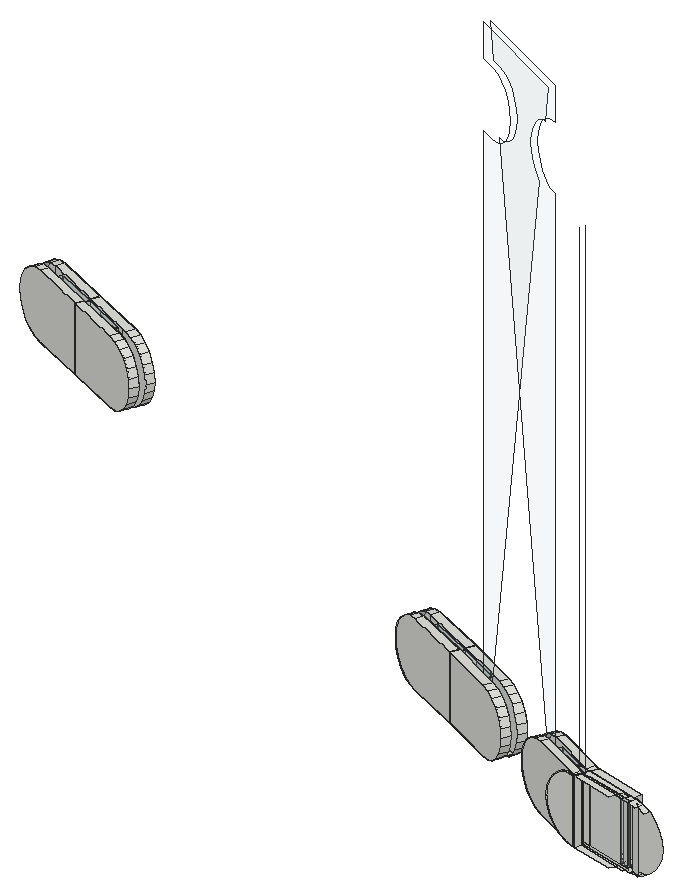
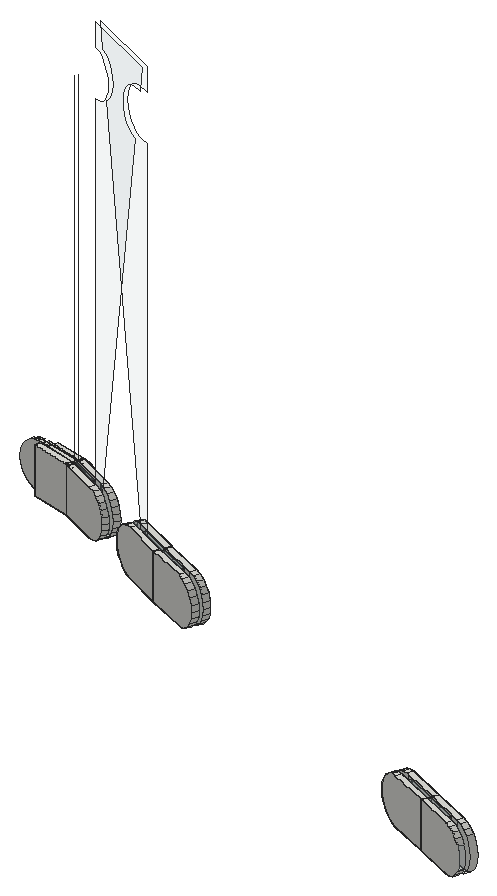
# SketchUp Ruby script. Lengths in inches.
U = 1.inch
M = Sketchup.active_model
def pt(a) = Geom::Point3d.new(a.map { |v| v * U })
def face(e, loops, mat)
  f = e.add_face(loops[0].map { |a| pt(a) })
  loops[1..].each { |l| e.add_face(l.map { |a| pt(a) }).erase! }
  f.material = f.back_material = mat if mat
  f
end
# faces: each face lists its corners as indices into pts; further lists are holes
def faces(e, pts, list, mat = nil) = list.each { |f| face(e, (f[0].is_a?(Array) ? f : [f]).map { |l| l.map { |i| pts[i] } }, mat) }
# xy, xz, yz: faces in a plane at the given z, y or x. An outline is a flat list of corners, or four numbers for a rectangle; further outlines are holes
def ring(l) = l.size == 4 ? [[l[0], l[1]], [l[2], l[1]], [l[2], l[3]], [l[0], l[3]]] : l.each_slice(2).to_a
def flat(e, list, mat, &to3) = list.each { |f| face(e, (f[0].is_a?(Array) ? f : [f]).map { |l| ring(l).map { |u, v| to3.(u, v) } }, mat) }
def xy(e, z, list, mat = nil) = flat(e, list, mat) { |x, y| [x, y, z] }
def xz(e, y, list, mat = nil) = flat(e, list, mat) { |x, z| [x, y, z] }
def yz(e, x, list, mat = nil) = flat(e, list, mat) { |y, z| [x, y, z] }
def lines(e, pts, list) = list.each { |a, b| e.add_line(pt(pts[a]), pt(pts[b])) }
# prism: a flat outline (further loops are holes) pulled along v
def prism(e, loops, v, mat = nil)
  f = face(e, loops, mat); d = Geom::Vector3d.new(v.map { |x| x * U })
  f.pushpull(f.normal.samedirection?(d) ? d.length : -d.length)
end
def box(e, o, s, mat = nil) = prism(e, [[o, [o[0] + s[0], o[1], o[2]], [o[0] + s[0], o[1] + s[1], o[2]], [o[0], o[1] + s[1], o[2]]]], [0, 0, s[2]], mat)
def at(x, y, z, deg = 0) = Geom::Transformation.translation(pt([x, y, z])) * Geom::Transformation.rotation(ORIGIN, Z_AXIS, deg.degrees)
def axes(o, x, y, z) = Geom::Transformation.new([*x, 0, *y, 0, *z, 0, *pt(o).to_a, 1])
def part(name) = M.definitions.add(name)
# library, detail: a bought-in or finely detailed component or shape, given as its bounding box
def library(name, o, s) = part(name).tap { |d| box(d.entities, o, s) }
def detail(e, o, s) = box(e.add_group.entities, o, s)
def put(e, d, t, mat = nil) = e.add_instance(d, t).tap { |i| i.material = mat if mat }
def group(e, t, mat = nil) = e.add_group.tap { |g| g.transformation = t; g.material = mat if mat }.entities
root = M.entities
M.materials.add("Glass_Safety_01").color = [204, 235, 244]
M.materials["Glass_Safety_01"].alpha = 0.1
xy(root,333,[[1023.371,1012.372,1021.983,1012.675,1022.025,1012.868,1023.251,1012.599,1023.444,1012.558],[1023.716,1012.498,1023.444,1012.558,1023.473,1012.632,1023.745,1012.572],[1023.965,1012.524,1023.94,1012.53,1023.97,1012.608,1023.982,1012.603],[1023.94,1012.53,1023.858,1012.548,1023.745,1012.572,1023.787,1012.68,1023.53,1012.78,1023.473,1012.632,1022.042,1012.945,1022.084,1013.137,1022.095,1013.134,1022.105,1013.13,1022.106,1013.132,1023.9,1012.74,1024.007,1012.717,1023.982,1012.603,1023.97,1012.608],[1023.444,1012.558,1023.251,1012.599,1022.025,1012.868,1022.042,1012.945,1023.473,1012.632],
  [1023.745,1012.572,1023.473,1012.632,1023.53,1012.78,1023.787,1012.68],[1021.983,1012.675,1021.876,1012.699,1021.879,1012.714,1021.903,1012.702,1022.02,1012.949,1022.042,1012.945,1022.025,1012.868],[1021.903,1012.702,1021.879,1012.714,1021.935,1012.968,1022.02,1012.949],[1021.879,1012.714,1020.123,1013.542,1020.24,1013.791,1022.021,1012.952,1022.02,1012.949,1021.935,1012.968],[1023.9,1012.74,1022.106,1013.132,1022.222,1013.379,1022.184,1013.397,1023.959,1013.009],
  [1022.105,1013.13,1022.095,1013.134,1022.106,1013.132],[1022.106,1013.132,1022.095,1013.134,1021.983,1013.1875,1022.035,1013.429,1022.184,1013.397,1022.222,1013.379],[1022.095,1013.134,1022.084,1013.137,1021.977,1013.16,1021.983,1013.1875],[1021.983,1013.1875,1020.324,1013.969,1020.442,1014.219,1022.184,1013.397,1022.035,1013.429],[1017.116,1014.96,1015.346,1015.795,1015.456,1016.048,1016.751,1015.437,1016.921,1015.357,1017.234,1015.209],
  [1017.318,1015.387,1016.835,1015.615,1015.537,1016.227,1015.655,1016.476,1017.435,1015.637],[1015.346,1015.795,1015.341,1015.797,1015.336,1015.8,1015.453,1016.049,1015.456,1016.048],[1015.336,1015.8,1013.541,1016.581,1013.651,1016.834,1015.453,1016.049],[1015.535,1016.228,1013.73,1017.014,1013.84,1017.267,1015.645,1016.481],[998.018,1023.342,996.213,1024.128,996.324,1024.38,997.958,1023.669,998.128,1023.594],
  [998.207,1023.775,998.037,1023.849,996.402,1024.561,996.512,1024.814,998.317,1024.028],[996.213,1024.128,994.409,1024.914,994.519,1025.167,996.324,1024.38],[996.402,1024.561,994.597,1025.347,994.707,1025.6,996.512,1024.814]])
xy(root,333.078,[[1023.858,1012.548,1023.745,1012.572,1023.787,1012.68,1023.879,1012.644],[1023.745,1012.572,1023.58,1012.608,1023.622,1012.801,1023.9,1012.74,1023.879,1012.644,1023.787,1012.68],[1023.58,1012.608,1022.319,1012.884,1022.361,1013.076,1023.622,1012.801],[1022.319,1012.884,1022.042,1012.945,1022.063,1013.041,1022.105,1013.13,1022.095,1013.134,1022.361,1013.076],[1022.021,1012.952,1020.597,1013.623,1020.681,1013.801,1022.095,1013.134,1022.084,1013.137,1022.063,1013.041],
  [1022.063,1013.041,1022.084,1013.137,1022.095,1013.134,1022.105,1013.13],[1016.878,1015.377,1016.751,1015.437,1015.456,1016.048,1015.495,1016.138,1015.537,1016.227,1016.835,1015.615,1016.962,1015.555],[1015.455,1016.048,1015.453,1016.049,1015.495,1016.138,1015.456,1016.048],[1015.453,1016.049,1014.012,1016.677,1014.091,1016.857,1015.535,1016.228,1015.495,1016.138],[997.767,1023.752,996.324,1024.38,996.402,1024.561,997.846,1023.932],
  [996.324,1024.38,994.88,1025.009,994.958,1025.19,996.402,1024.561]],"Glass_Safety_01")
xy(root,335.047,[[1023.858,1012.548,1023.879,1012.644,1023.787,1012.68,1023.745,1012.572],[1023.745,1012.572,1023.787,1012.68,1023.879,1012.644,1023.9,1012.74,1023.622,1012.801,1023.58,1012.608],[1023.58,1012.608,1023.622,1012.801,1022.361,1013.076,1022.319,1012.884],[1022.319,1012.884,1022.361,1013.076,1022.095,1013.134,1022.105,1013.13,1022.063,1013.041,1022.042,1012.945],[1022.021,1012.952,1022.063,1013.041,1022.084,1013.137,1022.095,1013.134,1020.681,1013.801,1020.597,1013.623],
  [1022.063,1013.041,1022.105,1013.13,1022.095,1013.134,1022.084,1013.137],[1016.878,1015.377,1016.962,1015.555,1016.835,1015.615,1015.537,1016.227,1015.495,1016.138,1015.456,1016.048,1016.751,1015.437],[1015.455,1016.048,1015.456,1016.048,1015.495,1016.138,1015.453,1016.049],[1015.453,1016.049,1015.495,1016.138,1015.535,1016.228,1014.091,1016.857,1014.012,1016.677],[997.767,1023.752,997.846,1023.932,996.402,1024.561,996.324,1024.38],
  [996.324,1024.38,996.402,1024.561,994.958,1025.19,994.88,1025.009]],"Glass_Safety_01")
xy(root,335.125,[[1023.371,1012.372,1023.444,1012.558,1023.251,1012.599,1022.025,1012.868,1021.983,1012.675],[1023.716,1012.498,1023.745,1012.572,1023.473,1012.632,1023.444,1012.558],[1023.965,1012.524,1023.982,1012.603,1023.97,1012.608,1023.94,1012.53],[1023.94,1012.53,1023.97,1012.608,1023.982,1012.603,1024.007,1012.717,1023.9,1012.74,1022.106,1013.132,1022.105,1013.13,1022.095,1013.134,1022.084,1013.137,1022.042,1012.945,1023.473,1012.632,1023.53,1012.78,1023.787,1012.68,1023.745,1012.572,1023.858,1012.548],[1023.444,1012.558,1023.473,1012.632,1022.042,1012.945,1022.025,1012.868,1023.251,1012.599],
  [1023.745,1012.572,1023.787,1012.68,1023.53,1012.78,1023.473,1012.632],[1021.983,1012.675,1022.025,1012.868,1022.042,1012.945,1022.02,1012.949,1021.903,1012.702,1021.879,1012.714,1021.876,1012.699],[1021.903,1012.702,1022.02,1012.949,1021.935,1012.968,1021.879,1012.714],[1021.879,1012.714,1021.935,1012.968,1022.02,1012.949,1022.021,1012.952,1020.24,1013.791,1020.123,1013.542],[1023.9,1012.74,1023.959,1013.009,1022.184,1013.397,1022.222,1013.379,1022.106,1013.132],
  [1022.105,1013.13,1022.106,1013.132,1022.095,1013.134],[1022.106,1013.132,1022.222,1013.379,1022.184,1013.397,1022.035,1013.429,1021.983,1013.1875,1022.095,1013.134],[1022.095,1013.134,1021.983,1013.1875,1021.977,1013.16,1022.084,1013.137],[1021.983,1013.1875,1022.035,1013.429,1022.184,1013.397,1020.442,1014.219,1020.324,1013.969],[1017.116,1014.96,1017.234,1015.209,1016.751,1015.437,1015.456,1016.048,1015.346,1015.795],
  [1017.318,1015.387,1017.435,1015.637,1015.655,1016.476,1015.537,1016.227,1016.835,1015.615],[1015.346,1015.795,1015.456,1016.048,1015.453,1016.049,1015.336,1015.8,1015.341,1015.797],[1015.336,1015.8,1015.453,1016.049,1013.651,1016.834,1013.541,1016.581],[1015.535,1016.228,1015.645,1016.481,1013.84,1017.267,1013.73,1017.014],[998.018,1023.342,998.128,1023.594,997.958,1023.669,996.324,1024.38,996.213,1024.128],
  [998.207,1023.775,998.317,1024.028,996.512,1024.814,996.402,1024.561,998.037,1023.849],[996.213,1024.128,996.324,1024.38,994.519,1025.167,994.409,1024.914],[996.402,1024.561,996.512,1024.814,994.707,1025.6,994.597,1025.347]])
p = [[1024.276,1012.658,333.036],[1024.526,1012.603,333.142],[1024.484,1012.411,333.142],[1024.234,1012.466,333.036],[1023.745,1012.572,335.125],[1023.858,1012.548,335.125],
  [1023.858,1012.548,335.047],[1023.745,1012.572,335.047],[1023.58,1012.608,335.047],[1023.58,1012.608,333.078],[1023.745,1012.572,333.078],[1023.858,1012.548,333.078],
  [1023.858,1012.548,333],[1023.745,1012.572,333],[1023.473,1012.632,333],[1022.042,1012.945,333],[1022.042,1012.945,333.078],[1022.319,1012.884,333.078],
  [1022.319,1012.884,335.047],[1022.042,1012.945,335.047],[1022.042,1012.945,335.125],[1023.473,1012.632,335.125],[1024.007,1012.717,333],[1023.9,1012.74,333],
  [1023.9,1012.74,333.078],[1023.9,1012.74,335.047],[1023.9,1012.74,335.125],[1024.007,1012.717,335.125],[1024.276,1012.658,335.089],[1024.526,1012.603,334.983],
  [1024.741,1012.556,334.814],[1024.906,1012.52,334.594],[1025.01,1012.497,334.338],[1025.046,1012.49,334.0625],[1025.01,1012.497,333.787],[1024.906,1012.52,333.531],
  [1024.741,1012.556,333.311],[1023.97,1012.608,333],[1023.97,1012.608,333.078],[1023.97,1012.608,335.047],[1023.97,1012.608,335.125],[1023.982,1012.603,335.125],
  [1024.227,1012.508,335.125],[1024.227,1012.508,333],[1023.982,1012.603,333],[1023.965,1012.524,333],[1021.903,1012.702,335.125],[1021.879,1012.714,335.125],
  [1020.123,1013.542,335.125],[1019.874,1013.659,335.089],[1019.642,1013.769,334.983],[1019.443,1013.863,334.814],[1019.29,1013.935,334.594],[1019.194,1013.98,334.338],
  [1019.161,1013.995,334.0625],[1019.194,1013.98,333.787],[1019.29,1013.935,333.531],[1019.443,1013.863,333.311],[1019.642,1013.769,333.142],[1019.874,1013.659,333.036],
  [1020.123,1013.542,333],[1021.879,1012.714,333],[1021.903,1012.702,333],[1021.876,1012.699,333],[1021.983,1012.675,333],[1021.983,1012.675,335.125],
  [1021.876,1012.699,335.125],[1021.607,1012.757,335.089],[1021.357,1012.812,334.983],[1021.141,1012.859,334.814],[1020.976,1012.895,334.594],[1020.873,1012.918,334.338],
  [1020.837,1012.926,334.0625],[1020.873,1012.918,333.787],[1020.976,1012.895,333.531],[1021.141,1012.859,333.311],[1021.357,1012.812,333.142],[1021.607,1012.757,333.036],
  [1021.666,1013.027,333.036],[1021.929,1012.969,333],[1021.935,1012.968,333],[1022.021,1012.952,333],[1022.021,1012.952,333.078],[1022.021,1012.952,335.047],
  [1022.021,1012.952,335.125],[1022.02,1012.949,335.125],[1022.02,1012.949,333],[1022.025,1012.868,335.125],[1022.025,1012.868,333],[1022.095,1013.134,333.078],
  [1022.361,1013.076,333.078],[1023.622,1012.801,333.078],[1022.106,1013.132,333],[1022.095,1013.134,333],[1022.084,1013.137,333],[1022.084,1013.137,333.078],
  [1023.787,1012.68,333.078],[1023.787,1012.68,333],[1023.53,1012.78,333],[1023.53,1012.78,335.125],[1023.787,1012.68,335.125],[1023.787,1012.68,335.047],
  [1023.959,1013.009,333],[1023.959,1013.009,335.125],[1021.415,1013.081,333.142],[1021.935,1012.968,335.125],[1022.063,1013.041,333.078],[1020.24,1013.791,333],
  [1020.24,1013.791,335.125],[1020.597,1013.623,335.047],[1020.597,1013.623,333.078],[1021.666,1013.027,335.089],[1021.929,1012.969,335.125],[1021.2,1013.128,333.311],
  [1021.035,1013.164,333.531],[1020.932,1013.187,333.787],[1020.896,1013.195,334.0625],[1020.932,1013.187,334.338],[1021.035,1013.164,334.594],[1021.2,1013.128,334.814],
  [1021.415,1013.081,334.983],[1022.184,1013.397,335.125],[1022.184,1013.397,333],[1022.035,1013.429,333],[1021.767,1013.488,333.036],[1021.516,1013.543,333.142],
  [1021.301,1013.59,333.311],[1021.136,1013.626,333.531],[1021.032,1013.649,333.787],[1020.997,1013.656,334.0625],[1021.032,1013.649,334.338],[1021.136,1013.626,334.594],
  [1021.301,1013.59,334.814],[1021.516,1013.543,334.983],[1021.767,1013.488,335.089],[1022.035,1013.429,335.125],[1021.983,1013.1875,335.125],[1020.324,1013.969,335.125],
  [1020.324,1013.969,333],[1021.983,1013.1875,333],[1022.105,1013.13,333],[1022.105,1013.13,333.078],[1020.681,1013.801,333.078],[1020.681,1013.801,335.047],
  [1022.095,1013.134,335.047],[1022.105,1013.13,335.047],[1022.105,1013.13,335.125],[1022.095,1013.134,335.125],[1022.084,1013.137,335.125],[1021.977,1013.16,335.125],
  [1021.977,1013.16,333],[1022.084,1013.137,335.047],[1022.222,1013.379,333],[1022.222,1013.379,335.125],[1022.106,1013.132,335.125],[1021.708,1013.219,333.036],
  [1021.97,1013.162,333],[1021.97,1013.162,335.125],[1021.708,1013.219,335.089],[1021.457,1013.274,334.983],[1021.242,1013.321,334.814],[1021.077,1013.357,334.594],
  [1020.974,1013.379,334.338],[1020.938,1013.387,334.0625],[1020.974,1013.379,333.787],[1021.077,1013.357,333.531],[1021.242,1013.321,333.311],[1021.457,1013.274,333.142],
  [1020.442,1014.219,333],[1020.193,1014.336,333.036],[1019.961,1014.445,333.142],[1019.762,1014.539,333.311],[1019.609,1014.611,333.531],[1019.513,1014.657,333.787],
  [1019.481,1014.672,334.0625],[1019.513,1014.657,334.338],[1019.609,1014.611,334.594],[1019.762,1014.539,334.814],[1019.961,1014.445,334.983],[1020.193,1014.336,335.089],
  [1020.442,1014.219,335.125],[1019.992,1013.909,333.036],[1019.76,1014.018,333.142],[1019.992,1013.909,335.089],[1019.76,1014.018,334.983],[1019.561,1014.112,334.814],
  [1019.408,1014.184,334.594],[1019.312,1014.229,334.338],[1019.279,1014.245,334.0625],[1019.312,1014.229,333.787],[1019.408,1014.184,333.531],[1019.561,1014.112,333.311],
  [1019.848,1014.194,334.985],[1020.15,1014.051,333.025],[1020.076,1014.087,335.089],[1020.076,1014.087,333.036],[1019.844,1014.196,333.142],[1019.645,1014.29,333.311],
  [1019.492,1014.362,333.531],[1019.396,1014.407,333.787],[1019.363,1014.423,334.0625],[1019.396,1014.407,334.338],[1019.492,1014.362,334.594],[1019.645,1014.29,334.814],
  [1019.844,1014.196,334.983],[1017.116,1014.96,335.125],[1015.346,1015.795,335.125],[1015.346,1015.795,333],[1017.116,1014.96,333],[1017.365,1014.843,333.036],
  [1017.597,1014.733,333.142],[1017.796,1014.639,333.311],[1017.949,1014.567,333.531],[1018.045,1014.522,333.787],[1018.078,1014.507,334.0625],[1018.045,1014.522,334.338],
  [1017.949,1014.567,334.594],[1017.796,1014.639,334.814],[1017.597,1014.733,334.983],[1017.365,1014.843,335.089],[1017.483,1015.092,333.036],[1017.714,1014.983,333.142],
  [1016.921,1015.357,333],[1017.234,1015.209,333],[1017.914,1014.889,333.311],[1018.066,1014.817,333.531],[1018.162,1014.771,333.787],[1018.195,1014.756,334.0625],
  [1018.162,1014.771,334.338],[1018.066,1014.817,334.594],[1017.914,1014.889,334.814],[1017.714,1014.983,334.983],[1017.483,1015.092,335.089],[1017.249,1015.202,335.123],
  [1017.234,1015.209,335.125],[1016.751,1015.437,335.125],[1015.456,1016.048,335.125],[1015.456,1016.048,335.047],[1015.456,1016.048,333.078],[1015.456,1016.048,333],
  [1016.751,1015.437,333],[1016.751,1015.437,333.078],[1016.751,1015.437,335.047],[1016.878,1015.377,335.047],[1016.878,1015.377,333.078],[1016.835,1015.615,335.125],
  [1016.835,1015.615,335.047],[1016.962,1015.555,335.047],[1016.962,1015.555,333.078],[1016.835,1015.615,333.078],[1016.835,1015.615,333],[1017.318,1015.387,333],
  [1017.567,1015.27,333.036],[1017.798,1015.161,333.142],[1017.998,1015.067,333.311],[1018.15,1014.995,333.531],[1018.246,1014.949,333.787],[1018.279,1014.934,334.0625],
  [1018.246,1014.949,334.338],[1018.15,1014.995,334.594],[1017.998,1015.067,334.814],[1017.798,1015.161,334.983],[1017.567,1015.27,335.089],[1017.318,1015.387,335.125],
  [1015.655,1016.476,335.125],[1017.435,1015.637,335.125],[1017.684,1015.519,335.089],[1017.916,1015.41,334.983],[1018.115,1015.316,334.814],[1018.268,1015.244,334.594],
  [1018.364,1015.199,334.338],[1018.397,1015.183,334.0625],[1018.364,1015.199,333.787],[1018.268,1015.244,333.531],[1018.115,1015.316,333.311],[1017.916,1015.41,333.142],
  [1017.684,1015.519,333.036],[1017.435,1015.637,333],[1015.655,1016.476,333],[1015.537,1016.227,333],[1015.537,1016.227,333.078],[1015.341,1015.797,335.125],
  [1015.336,1015.8,335.125],[1013.541,1016.581,335.125],[1013.289,1016.691,335.089],[1013.054,1016.793,334.983],[1012.852,1016.881,334.814],[1012.697,1016.949,334.594],
  [1012.6,1016.991,334.338],[1012.567,1017.006,334.0625],[1012.6,1016.991,333.787],[1012.697,1016.949,333.531],[1012.852,1016.881,333.311],[1013.054,1016.793,333.142],
  [1013.289,1016.691,333.036],[1013.541,1016.581,333],[1015.336,1015.8,333],[1015.341,1015.797,333],[1015.453,1016.049,333.078],[1015.453,1016.049,333],
  [1015.453,1016.049,335.125],[1015.453,1016.049,335.047],[1013.651,1016.834,335.125],[1014.012,1016.677,335.047],[1014.012,1016.677,333.078],[1013.651,1016.834,333],
  [1013.399,1016.944,333.036],[1013.164,1017.046,333.142],[1012.962,1017.134,333.311],[1012.807,1017.201,333.531],[1012.71,1017.244,333.787],[1012.677,1017.258,334.0625],
  [1012.71,1017.244,334.338],[1012.807,1017.201,334.594],[1012.962,1017.134,334.814],[1013.164,1017.046,334.983],[1013.399,1016.944,335.089],[1015.455,1016.048,333.078],
  [1015.535,1016.228,335.125],[1013.73,1017.014,335.125],[1013.73,1017.014,333],[1015.535,1016.228,333],[1015.535,1016.228,333.078],[1014.091,1016.857,333.078],
  [1014.091,1016.857,335.047],[1015.535,1016.228,335.047],[1015.645,1016.481,333],[1015.645,1016.481,335.125],[1015.537,1016.227,335.047],[1015.537,1016.227,335.125],
  [1013.84,1017.267,335.125],[1013.84,1017.267,333],[1013.588,1017.377,333.036],[1013.353,1017.479,333.142],[1013.151,1017.567,333.311],[1012.996,1017.635,333.531],
  [1012.898,1017.677,333.787],[1012.865,1017.691,334.0625],[1012.898,1017.677,334.338],[1012.996,1017.635,334.594],[1013.151,1017.567,334.814],[1013.353,1017.479,334.983],
  [1013.588,1017.377,335.089],[1013.478,1017.124,333.036],[1013.242,1017.226,333.142],[1013.041,1017.314,333.311],[1012.886,1017.382,333.531],[1012.788,1017.424,333.787],
  [1012.755,1017.439,334.0625],[1012.788,1017.424,334.338],[1012.886,1017.382,334.594],[1013.041,1017.314,334.814],[1013.242,1017.226,334.983],[1013.478,1017.124,335.089],
  [998.018,1023.342,335.125],[996.213,1024.128,335.125],[996.213,1024.128,333],[998.018,1023.342,333],[998.27,1023.232,333.036],[998.506,1023.13,333.142],
  [998.707,1023.042,333.311],[998.862,1022.974,333.531],[998.96,1022.932,333.787],[998.993,1022.917,334.0625],[998.96,1022.932,334.338],[998.862,1022.974,334.594],
  [998.707,1023.042,334.814],[998.506,1023.13,334.983],[998.27,1023.232,335.089],[998.381,1023.485,333.036],[998.616,1023.382,333.142],[998.128,1023.594,333],
  [997.958,1023.669,333],[997.958,1023.669,335.125],[998.128,1023.594,335.125],[998.381,1023.485,335.089],[998.616,1023.382,334.983],[998.817,1023.294,334.814],
  [998.972,1023.227,334.594],[999.07,1023.184,334.338],[999.103,1023.17,334.0625],[999.07,1023.184,333.787],[998.972,1023.227,333.531],[998.817,1023.294,333.311],
  [998.207,1023.775,335.125],[998.037,1023.849,335.125],[998.037,1023.849,333],[998.207,1023.775,333],[998.459,1023.665,333.036],[998.694,1023.563,333.142],
  [998.896,1023.475,333.311],[999.051,1023.407,333.531],[999.148,1023.365,333.787],[999.181,1023.35,334.0625],[999.148,1023.365,334.338],[999.051,1023.407,334.594],
  [998.896,1023.475,334.814],[998.694,1023.563,334.983],[998.459,1023.665,335.089],[996.512,1024.814,335.125],[998.317,1024.028,335.125],[998.569,1023.918,335.089],
  [998.804,1023.815,334.983],[999.006,1023.727,334.814],[999.161,1023.66,334.594],[999.258,1023.618,334.338],[999.291,1023.603,334.0625],[999.258,1023.618,333.787],
  [999.161,1023.66,333.531],[999.006,1023.727,333.311],[998.804,1023.815,333.142],[998.569,1023.918,333.036],[998.317,1024.028,333],[996.512,1024.814,333],
  [996.324,1024.38,335.125],[996.324,1024.38,333],[996.324,1024.38,333.078],[997.767,1023.752,333.078],[997.767,1023.752,335.047],[996.324,1024.38,335.047],
  [996.402,1024.561,333],[996.402,1024.561,335.125],[996.402,1024.561,335.047],[997.846,1023.932,335.047],[997.846,1023.932,333.078],[996.402,1024.561,333.078],
  [994.409,1024.914,335.125],[994.156,1025.024,335.089],[993.921,1025.126,334.983],[993.72,1025.214,334.814],[993.565,1025.281,334.594],[993.467,1025.324,334.338],
  [993.434,1025.338,334.0625],[993.467,1025.324,333.787],[993.565,1025.281,333.531],[993.72,1025.214,333.311],[993.921,1025.126,333.142],[994.156,1025.024,333.036],
  [994.409,1024.914,333],[994.519,1025.167,333],[994.519,1025.167,335.125],[994.88,1025.009,335.047],[994.88,1025.009,333.078],[994.597,1025.347,335.125],
  [994.597,1025.347,333],[994.958,1025.19,333.078],[994.958,1025.19,335.047],[994.707,1025.6,335.125],[994.707,1025.6,333],[994.455,1025.71,333.036],
  [994.22,1025.812,333.142],[994.018,1025.9,333.311],[993.863,1025.967,333.531],[993.766,1026.01,333.787],[993.733,1026.024,334.0625],[993.766,1026.01,334.338],
  [993.863,1025.967,334.594],[994.018,1025.9,334.814],[994.22,1025.812,334.983],[994.455,1025.71,335.089],[994.267,1025.276,333.036],[994.031,1025.379,333.142],
  [994.267,1025.276,335.089],[994.031,1025.379,334.983],[993.83,1025.467,334.814],[993.675,1025.534,334.594],[993.577,1025.577,334.338],[993.544,1025.591,334.0625],
  [993.577,1025.577,333.787],[993.675,1025.534,333.531],[993.83,1025.467,333.311],[994.345,1025.457,333.036],[994.11,1025.559,333.142],[993.908,1025.647,333.311],
  [993.753,1025.715,333.531],[993.656,1025.757,333.787],[993.623,1025.771,334.0625],[993.656,1025.757,334.338],[993.753,1025.715,334.594],[993.908,1025.647,334.814],
  [994.11,1025.559,334.983],[994.345,1025.457,335.089],[1023.879,1012.644,333.078],[1023.879,1012.644,335.047],[1023.622,1012.801,335.047],[1022.361,1013.076,335.047],
  [1022.063,1013.041,335.047],[1015.455,1016.048,335.047],[1015.495,1016.138,335.047],[1015.495,1016.138,333.078],[1024.234,1012.466,335.089],[1024.484,1012.411,334.983],
  [1020.324,1013.969,351.283],[1017.333,1015.38,351.285],[1017.567,1015.27,351.319],[1017.798,1015.161,351.425],[1017.998,1015.067,351.594],[1018.15,1014.995,351.814],
  [1018.246,1014.949,352.071],[1018.279,1014.934,352.346],[1018.246,1014.949,352.621],[1018.15,1014.995,352.877],[1017.998,1015.067,353.098],[1017.798,1015.161,353.267],
  [1017.567,1015.27,353.373],[1017.318,1015.387,353.409],[1017.005,1015.535,353.409],[1016.835,1015.615,354.511],[1020.324,1013.969,354.511],[1020.324,1013.969,353.409],
  [1020.076,1014.087,353.373],[1019.844,1014.196,353.267],[1019.645,1014.29,353.098],[1019.492,1014.362,352.877],[1019.396,1014.407,352.621],[1019.363,1014.423,352.346],
  [1019.396,1014.407,352.071],[1019.492,1014.362,351.814],[1019.645,1014.29,351.594],[1019.844,1014.196,351.425],[1020.076,1014.087,351.319],[1023.965,1012.524,335.125],
  [1024.217,1012.389,335.089],[1023.948,1012.447,335.125],[1021.935,1012.968,351.283],[1021.928,1012.969,351.284],[1021.971,1013.161,351.284],[1021.977,1013.16,351.283],
  [1019.764,1014.016,351.423],[1019.76,1014.018,351.425],[1019.561,1014.112,351.594],[1019.408,1014.184,351.814],[1019.312,1014.229,352.071],[1019.279,1014.245,352.346],
  [1019.312,1014.229,352.621],[1019.408,1014.184,352.877],[1019.561,1014.112,353.098],[1019.76,1014.018,353.267],[1019.992,1013.909,353.373],[1020.066,1013.873,353.384],
  [1020.24,1013.791,354.511],[1016.751,1015.437,354.511],[1016.751,1015.437,353.409],[1017.234,1015.209,353.409],[1017.483,1015.092,353.373],[1017.714,1014.983,353.267],
  [1017.914,1014.889,353.098],[1018.066,1014.817,352.877],[1018.162,1014.771,352.621],[1018.195,1014.756,352.346],[1018.162,1014.771,352.071],[1018.066,1014.817,351.814],
  [1017.914,1014.889,351.594],[1017.714,1014.983,351.425],[1017.483,1015.092,351.319],[1017.234,1015.209,351.283],[1016.751,1015.437,351.283]]
faces(root,p,[[0,1,2,3],[4,5,6,7,8,9,10,11,12,13,14,15,16,17,18,19,20,21],[22,23,24,25,26,27,28,29,30,31,32,33,34,35,36,1,0],[37,38,39,40,41,42,43,44],[22,0,3,45,44],[46,47,48,49,50,51,52,53,54,55,56,57,58,59,60,61,62],[63,64,65,66,67,68,69,70,71,72,73,74,75,76,77],[78,79,80,61,63,77],
  [81,82,83,84,85,46,62,86],[87,65,64,88],[89,90,91,24,23,92,93,94,95],[96,97,98,99,100,101],[24,23,102,103,26,25],[104,78,77,76],[86,80,105,85,20,19,16,15],[15,16,19,20,87,88],
  [95,106,16,15,94],[81,107,108,84,83,109,110,82],[111,112,79,78,104,113,114,115,116,117,118,119,120],[121,103,102,122,123,124,125,126,127,128,129,130,131,132,133,134,135],[136,137,138,139,93,140,141,89,142,143,144,145,146,147],[148,149,150,94,95,151],[141,140,92,152,153,154,146,145],[155,156,157,158,159,160,161,162,163,164,165,166,167],
  [155,167,125,124],[156,155,124,123,139,150],[149,157,156,150],[121,153,152,122,168,169,170,171,172,173,174,175,176,177,178,179,180],[181,107,60,59],[182,181,59,58],[193,195,169,168,138],[195,196,170,169],
  [205,206,207,208,209,210,211,212,213,214,215,216,217,218,219],[220,221,210,209],[223,220,209,208],[264,265,266,267,268,269,270,271,272,273,274,275,276,277,278],[253,252,276,275],[252,251,277,276],[279,250,249,280],[206,281,282,283,284,285,286,287,288,289,290,291,292,293,294,295,296,297,207],
  [297,207,206,281,282,296],[298,299,296,282,300,301],[239,238,237,236,206,207],[302,300,301,303,304,298,299,305,306,307,308,309,310,311,312,313,314,315,316],[239,299,298,317,238],[300,236,237,238,239,299,298,301],[318,319,320,321,322,323,324,325],[322,321,326,327,318,325],
  [279,280,328,329,264,278],[330,327,326,331,332,333,334,335,336,337,338,339,340,341,342],[306,305,295,294],[307,306,294,293],[320,343,332,331],[343,344,333,332],[354,355,356,357,358,359,360,361,362,363,364,365,366,367,368],[369,370,359,358],
  [371,369,358,357],[371,372,373,374,375,376,377,378,379,380,381,382,383,370,369],[384,385,386,387,388,389,390,391,392,393,394,395,396,397,398],[399,400,401,402,403,404,405,406,407,408,409,410,411,412,413],[389,388,411,410],[414,373,372,415,416,417,418,419],[388,387,412,411],[420,386,385,421,422,423,424,425],
  [355,426,427,428,429,430,431,432,433,434,435,436,437,438,356],[416,415,356,355,414,419],[415,439,440,414,419,441,442,416],[421,443,444,420,425,445,446,422],[420,425,422,421,399,413],[447,399,413,448,449,450,451,452,453,454,455,456,457,458,459],[460,439,438,437],[461,460,437,436],
  [444,471,449,448],[471,472,450,449],[113,104,76,75],[106,486,19,16],[16,19,18,17],[167,166,126,125],[191,182,58,57],[196,197,171,170],
  [221,224,211,210],[254,253,275,274],[308,307,293,292],[344,345,334,333],[370,383,360,359],[390,389,410,409],[472,473,451,450],[114,113,75,74],
  [166,165,127,126],[190,191,57,56],[197,198,172,171],[224,225,212,211],[255,254,274,273],[309,308,292,291],[345,346,335,334],[383,382,361,360],
  [391,390,409,408],[473,474,452,451],[115,114,74,73],[165,164,128,127],[189,190,56,55],[198,199,173,172],[225,226,213,212],[256,255,273,272],
  [310,309,291,290],[346,347,336,335],[382,381,362,361],[392,391,408,407],[116,115,73,72],[164,163,129,128],[188,189,55,54],[199,200,174,173],
  [226,227,214,213],[257,256,272,271],[311,310,290,289],[347,348,337,336],[381,380,363,362],[393,392,407,406],[117,116,72,71],[163,162,130,129],
  [187,188,54,53],[200,201,175,174],[227,228,215,214],[258,257,271,270],[312,311,289,288],[348,349,338,337],[380,379,364,363],[394,393,406,405],
  [118,117,71,70],[162,161,131,130],[186,187,53,52],[201,202,176,175],[228,229,216,215],[259,258,270,269],[313,312,288,287],[349,350,339,338],
  [379,378,365,364],[395,394,405,404],[119,118,70,69],[161,160,132,131],[185,186,52,51],[202,203,177,176],[229,230,217,216],[260,259,269,268],
  [314,313,287,286],[350,351,340,339],[378,377,366,365],[396,395,404,403],[478,479,457,456],[120,119,69,68],[160,159,133,132],[184,185,51,50],
  [203,204,178,177],[230,231,218,217],[261,260,268,267],[315,314,286,285],[351,352,341,340],[377,376,367,366],[397,396,403,402],[463,464,429,428],
  [479,480,458,457],[29,28,490,491],[25,484,485,144,151,148,147,154,26],[111,120,68,67],[20,19,486,151,148],[159,158,134,133],[183,184,50,49],[192,194,179,178,204],
  [231,232,219,218],[262,261,267,266],[328,246,245,329],[487,301,300,236,237],[316,315,285,284],[352,353,342,341],[376,375,368,367],[398,397,402,401],
  [462,463,428,427],[480,481,459,458],[521,41,27,28,490,522,523],[105,112,111,67,66,47],[157,149,136,135,134,158],[108,183,49,48],[194,137,180,179],[233,234,205,219,232],
  [263,262,266,265],[302,316,284,283],[353,319,330,342],[375,374,354,368],[384,398,401,400],[440,462,427,426],[481,443,447,459]])
faces(root,p,[[112,79,80,105],[107,108,183,184,185,186,187,188,189,190,191,182,181],[192,193,138,137,194],[192,193,195,196,197,198,199,200,201,202,203,204],[[222,223,220,221,224,225,226,227,228,229,230,231,232,233,234,235,236,237,238,239,240],[241,242,243,244]],[233,222,223,220,221,224,225,226,227,228,229,230,231,232],[245,246,247,248,249,250,251,252,253,254,255,256,257,258,259,260,261,262,263],[222,233,234,235,242,243,244,241,240],
  [305,302,316,315,314,313,312,311,310,309,308,307,306],[319,320,343,344,345,346,347,348,349,350,351,352,353],[439,440,462,463,464,465,466,467,468,469,470,461,460],[443,444,471,472,473,474,475,476,477,478,479,480,481],[8,7,6,11,10,9],[482,483,6,11],[17,9,8,18],[91,484,8,9],
  [101,483,482,96],[483,482,24,25],[38,482,483,39],[24,91,484,25],[91,90,485,484],[90,17,18,485],[82,110,109,83],[106,486,83,82],
  [106,95,151,486],[486,106,141,145],[89,141,145,144,143,142],[144,485,90,89,95,151],[109,143,142,110],[238,241,242,237],[242,241,244,243],[248,247,243,244],
  [246,328,280,249],[249,246,247,248],[303,301,298,304],[317,298,301,487,237,238],[301,488,489,298],[489,488,237,238],[488,489,322,325],[280,489,488,328],
  [323,322,325,324],[323,304,303,324],[417,416,419,418],[424,423,418,417],[425,424,423,422],[416,442,441,419],[425,416,419,422],[445,425,422,446],
  [442,441,446,445],[492,137,194,192,493,494,495,496,497,498,499,500,501,502,503,504,505,506,507,508,509,510,511,512,513,514,515,516,517,518,519,520],[112,524,525],[524,112,105],[526,149,157],[149,526,527],[233,528,529,530,531,532,533,534,535,536,537,538,539,540,541,542,543,544,545,546,547,548,549,550,551,552,553,554,555,556,235,234]],"Glass_Safety_01")
